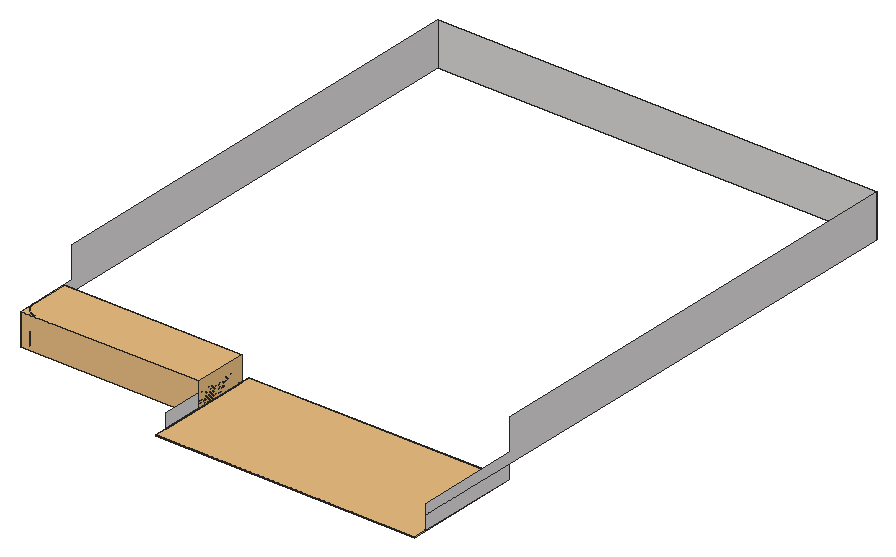
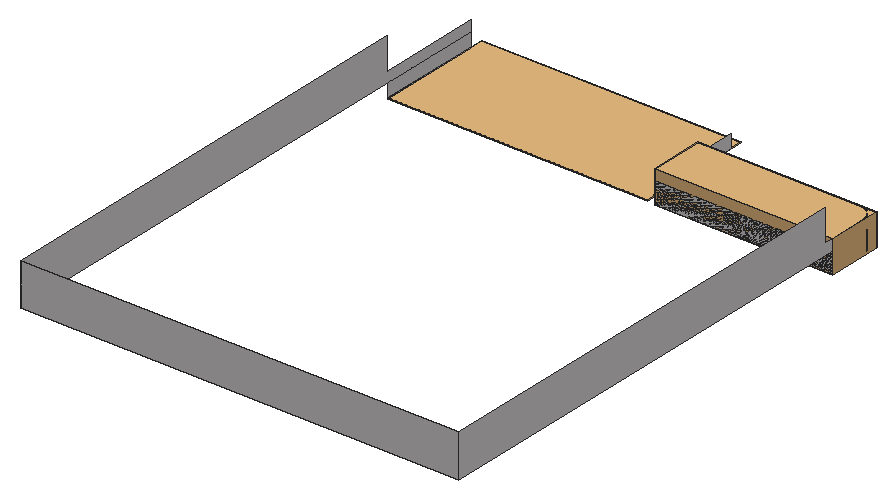
# SketchUp Ruby script. Lengths in inches.
U = 1.inch
M = Sketchup.active_model
def pt(a) = Geom::Point3d.new(a.map { |v| v * U })
def face(e, loops, mat)
  f = e.add_face(loops[0].map { |a| pt(a) })
  loops[1..].each { |l| e.add_face(l.map { |a| pt(a) }).erase! }
  f.material = f.back_material = mat if mat
  f
end
# faces: each face lists its corners as indices into pts; further lists are holes
def faces(e, pts, list, mat = nil) = list.each { |f| face(e, (f[0].is_a?(Array) ? f : [f]).map { |l| l.map { |i| pts[i] } }, mat) }
# xy, xz, yz: faces in a plane at the given z, y or x. An outline is a flat list of corners, or four numbers for a rectangle; further outlines are holes
def ring(l) = l.size == 4 ? [[l[0], l[1]], [l[2], l[1]], [l[2], l[3]], [l[0], l[3]]] : l.each_slice(2).to_a
def flat(e, list, mat, &to3) = list.each { |f| face(e, (f[0].is_a?(Array) ? f : [f]).map { |l| ring(l).map { |u, v| to3.(u, v) } }, mat) }
def xy(e, z, list, mat = nil) = flat(e, list, mat) { |x, y| [x, y, z] }
def xz(e, y, list, mat = nil) = flat(e, list, mat) { |x, z| [x, y, z] }
def yz(e, x, list, mat = nil) = flat(e, list, mat) { |y, z| [x, y, z] }
def lines(e, pts, list) = list.each { |a, b| e.add_line(pt(pts[a]), pt(pts[b])) }
# prism: a flat outline (further loops are holes) pulled along v
def prism(e, loops, v, mat = nil)
  f = face(e, loops, mat); d = Geom::Vector3d.new(v.map { |x| x * U })
  f.pushpull(f.normal.samedirection?(d) ? d.length : -d.length)
end
def box(e, o, s, mat = nil) = prism(e, [[o, [o[0] + s[0], o[1], o[2]], [o[0] + s[0], o[1] + s[1], o[2]], [o[0], o[1] + s[1], o[2]]]], [0, 0, s[2]], mat)
def at(x, y, z, deg = 0) = Geom::Transformation.translation(pt([x, y, z])) * Geom::Transformation.rotation(ORIGIN, Z_AXIS, deg.degrees)
def axes(o, x, y, z) = Geom::Transformation.new([*x, 0, *y, 0, *z, 0, *pt(o).to_a, 1])
def part(name) = M.definitions.add(name)
# library, detail: a bought-in or finely detailed component or shape, given as its bounding box
def library(name, o, s) = part(name).tap { |d| box(d.entities, o, s) }
def detail(e, o, s) = box(e.add_group.entities, o, s)
def put(e, d, t, mat = nil) = e.add_instance(d, t).tap { |i| i.material = mat if mat }
def group(e, t, mat = nil) = e.add_group.tap { |g| g.transformation = t; g.material = mat if mat }.entities
root = M.entities
M.materials.add("Outer Light - 1").color = [251, 216, 141]
M.materials.add("[Quartz Light Brown]").color = [215, 212, 212]
M.materials.add("[Wood Cherry Original]").color = [152, 86, 42]
c1 = library("Group\#15",[-0.75,-0.75,0],[293.5,131.75,1])
c2 = library("Group\#45",[-0.5,-0.5,0],[201.5,61.5,36])
xy(root,360,[[[17.76,205,17.53,205.01,17.29,205.01,17.06,205.02,16.82,205.04,16.59,205.06,16.35,205.08,16.12,205.1,15.88,205.125,15.65,205.15,15.42,205.1875,15.18,205.22,14.72,205.3,14.49,205.35,14.26,205.39,14.03,205.44,13.8,205.5,13.57,205.55,13.34,205.61,13.11,205.68,12.89,205.74,12.66,205.81,12.4375,205.88,12.21,205.96,11.99,206.03,11.77,206.11,11.55,206.2,11.33,206.28,10.89,206.46,10.68,206.56,10.46,206.65,10.25,206.75,10.04,206.86,9.83,206.96,9.41,207.18,9.2,207.3,9,207.41,8.6,207.65,8.39,207.78,8.2,207.9,8,208.03,7.8,208.17,7.61,208.3,7.42,208.4375,7.23,208.58,7.04,208.72,6.86,208.86,6.67,209.01,6.49,209.16,6.31,209.3125,6.13,209.47,5.96,209.625,5.78,209.78,5.61,209.94,5.44,210.11,5.27,210.27,5.11,210.44,4.94,210.61,4.78,210.78,4.625,210.96,4.47,211.13,4.3125,211.31,4.16,211.49,4.01,211.67,3.86,211.86,3.72,212.04,3.58,212.23,3.4375,212.42,3.3,212.61,3.17,212.8,3.03,213,2.9,213.2,2.78,213.39,2.65,213.6,2.41,214,2.3,214.2,2.18,214.41,1.96,214.83,1.86,215.04,1.75,215.25,1.65,215.46,1.56,215.68,1.46,215.89,1.28,216.33,1.2,216.55,1.11,216.77,1.03,216.99,0.96,217.21,0.88,217.4375,0.81,217.66,0.74,217.89,0.68,218.11,0.61,218.34,0.55,218.57,0.5,218.8,0.44,219.03,0.39,219.26,0.35,219.49,0.3,219.72,0.22,220.18,0.1875,220.42,0.15,220.65,0.125,220.88,0.1,221.12,0.08,221.35,0.06,221.59,0.04,221.82,0.02,222.06,0.01,222.29,0.01,222.53,0,222.76,0,266,201,266,201,205],[17.79,207,199,207,199,264,2,264,2,222.79,2.01,222.58,2.01,222.37,2.03,221.95,2.05,221.74,2.07,221.54,2.11,221.12,2.17,220.7,2.2,220.5,2.23,220.29,2.27,220.08,2.31,219.88,2.35,219.67,2.39,219.47,2.44,219.26,2.49,219.0625,2.55,218.86,2.6,218.66,2.78,218.06,2.99,217.46,3.0625,217.27,3.14,217.07,3.22,216.88,3.3,216.68,3.38,216.49,3.65,215.92,3.74,215.74,3.84,215.55,3.9375,215.37,4.04,215.18,4.14,215,4.47,214.46,4.58,214.29,4.7,214.11,4.8125,213.9375,4.93,213.77,5.06,213.6,5.18,213.43,5.31,213.26,5.43,213.09,5.57,212.93,5.83,212.61,6.11,212.29,6.39,211.99,6.54,211.84,6.6875,211.6875,6.84,211.54,6.99,211.39,7.29,211.11,7.61,210.83,7.93,210.57,8.09,210.43,8.26,210.31,8.43,210.18,8.6,210.06,8.77,209.93,8.9375,209.8125,9.11,209.7,9.29,209.58,9.46,209.47,10,209.14,10.18,209.04,10.37,208.9375,10.55,208.84,10.74,208.74,10.92,208.65,11.49,208.38,11.68,208.3,11.88,208.22,12.07,208.14,12.27,208.0625,12.46,207.99,13.06,207.78,13.66,207.6,13.86,207.55,14.0625,207.49,14.26,207.44,14.47,207.39,14.67,207.35,14.88,207.31,15.08,207.27,15.29,207.23,15.5,207.2,15.7,207.17,16.12,207.11,16.54,207.07,16.74,207.05,16.95,207.03,17.37,207.01,17.58,207.01]]],"[Quartz Light Brown]")
xy(root,366,[[17.79,207,17.58,207.01,17.37,207.01,16.95,207.03,16.74,207.05,16.54,207.07,16.12,207.11,15.7,207.17,15.5,207.2,15.29,207.23,15.08,207.27,14.88,207.31,14.67,207.35,14.47,207.39,14.26,207.44,14.0625,207.49,13.86,207.55,13.66,207.6,13.06,207.78,12.46,207.99,12.27,208.0625,12.07,208.14,11.88,208.22,11.68,208.3,11.49,208.38,10.92,208.65,10.74,208.74,10.55,208.84,10.37,208.9375,10.18,209.04,10,209.14,9.46,209.47,9.29,209.58,9.11,209.7,8.9375,209.8125,8.77,209.93,8.6,210.06,8.43,210.18,8.26,210.31,8.09,210.43,7.93,210.57,7.61,210.83,7.29,211.11,6.99,211.39,6.84,211.54,6.6875,211.6875,6.54,211.84,6.39,211.99,6.11,212.29,5.83,212.61,5.57,212.93,5.43,213.09,5.31,213.26,5.18,213.43,5.06,213.6,4.93,213.77,4.8125,213.9375,4.7,214.11,4.58,214.29,4.47,214.46,4.14,215,4.04,215.18,3.9375,215.37,3.84,215.55,3.74,215.74,3.65,215.92,3.38,216.49,3.3,216.68,3.22,216.88,3.14,217.07,3.0625,217.27,2.99,217.46,2.78,218.06,2.6,218.66,2.55,218.86,2.49,219.0625,2.44,219.26,2.39,219.47,2.35,219.67,2.31,219.88,2.27,220.08,2.23,220.29,2.2,220.5,2.17,220.7,2.11,221.12,2.07,221.54,2.05,221.74,2.03,221.95,2.01,222.37,2.01,222.58,2,222.79,2,264,199,264,199,207]],"[Quartz Light Brown]")
xz(root,207,[[17.79,360,18,366],[18,360,199,366]],"[Quartz Light Brown]")
xz(root,207.01,[[17.37,360,17.58,366]],"[Quartz Light Brown]")
xz(root,264,[[2,360,199,366]],"[Quartz Light Brown]")
xz(root,266,[[0,360,201,384]],"[Quartz Light Brown]")
xz(root,794,[[0,384,495,432]],"[Quartz Light Brown]")
yz(root,0,[[222.76,360,223,396],[223,360,266,396],[266,384,266,396,276.5,396,276.5,432,794,432,794,384]],"[Quartz Light Brown]")
yz(root,0.01,[[222.29,360,222.53,396]],"[Quartz Light Brown]")
yz(root,2,[[222.79,360,223,366],[223,360,264,366]],"[Quartz Light Brown]")
yz(root,2.01,[[222.37,360,222.58,366]],"[Quartz Light Brown]")
yz(root,199,[[207,360,264,366]],"[Quartz Light Brown]")
yz(root,201,[[205,360,266,384],[158,369,266,384]],"[Quartz Light Brown]")
yz(root,202,[[158,368,266,369]],"[Quartz Light Brown]")
yz(root,494,[[158,368,275,369]],"[Quartz Light Brown]")
yz(root,495,[[158,369,275,384],[158,384,794,384,794,432,276.5,432,276.5,396,158,396]],"[Quartz Light Brown]")
p = [[15.18,205.22,396],[14.95,205.26,396],[14.95,205.26,360],[15.18,205.22,360],[15.42,205.1875,396],[15.42,205.1875,360],
  [14.49,205.35,396],[14.26,205.39,396],[14.26,205.39,360],[14.49,205.35,360],[14.72,205.3,396],[14.72,205.3,360],
  [14.03,205.44,396],[13.8,205.5,396],[13.8,205.5,360],[14.03,205.44,360],[13.57,205.55,396],[13.57,205.55,360],
  [13.34,205.61,396],[13.11,205.68,396],[13.11,205.68,360],[13.34,205.61,360],[12.89,205.74,396],[12.66,205.81,396],
  [12.66,205.81,360],[12.89,205.74,360],[12.4375,205.88,396],[12.4375,205.88,360],[12.21,205.96,396],[12.21,205.96,360],
  [11.99,206.03,396],[11.77,206.11,396],[11.77,206.11,360],[11.99,206.03,360],[11.55,206.2,396],[11.55,206.2,360],
  [11.33,206.28,396],[11.33,206.28,360],[11.11,206.37,396],[11.11,206.37,360],[10.89,206.46,396],[10.89,206.46,360],
  [10.68,206.56,396],[10.68,206.56,360],[10.46,206.65,396],[10.46,206.65,360],[10.25,206.75,396],[10.25,206.75,360],
  [10.04,206.86,396],[10.04,206.86,360],[9.83,206.96,396],[9.83,206.96,360],[9.62,207.07,396],[9.62,207.07,360],
  [16.74,207.05,360],[16.54,207.07,360],[16.54,207.07,366],[16.74,207.05,366],[16.95,207.03,360],[16.95,207.03,366],
  [17.16,207.02,360],[17.16,207.02,366],[17.37,207.01,360],[17.37,207.01,366],[17.79,207,360],[17.58,207.01,360],
  [17.58,207.01,366],[17.79,207,366],[9.41,207.18,396],[9.41,207.18,360],[15.91,207.14,360],[15.7,207.17,360],
  [15.7,207.17,366],[15.91,207.14,366],[16.12,207.11,360],[16.12,207.11,366],[16.33,207.09,360],[16.33,207.09,366],
  [9.2,207.3,396],[9.2,207.3,360],[15.29,207.23,360],[15.08,207.27,360],[15.08,207.27,366],[15.29,207.23,366],
  [15.5,207.2,360],[15.5,207.2,366],[9,207.41,396],[9,207.41,360],[14.67,207.35,360],[14.47,207.39,360],
  [14.47,207.39,366],[14.67,207.35,366],[14.88,207.31,360],[14.88,207.31,366],[8.8,207.53,396],[8.8,207.53,360],
  [14.26,207.44,360],[14.0625,207.49,360],[14.0625,207.49,366],[14.26,207.44,366],[8.6,207.65,396],[8.6,207.65,360],
  [13.86,207.55,360],[13.66,207.6,360],[13.66,207.6,366],[13.86,207.55,366],[13.46,207.66,360],[13.46,207.66,366],
  [8.39,207.78,396],[8.39,207.78,360],[13.26,207.72,360],[13.06,207.78,360],[13.06,207.78,366],[13.26,207.72,366],
  [8.2,207.9,396],[8.2,207.9,360],[12.86,207.85,360],[12.66,207.92,360],[12.66,207.92,366],[12.86,207.85,366],
  [8,208.03,396],[8,208.03,360],[12.46,207.99,360],[12.46,207.99,366],[7.8,208.17,396],[7.8,208.17,360],
  [12.27,208.0625,360],[12.27,208.0625,366],[12.07,208.14,360],[11.88,208.22,360],[11.88,208.22,366],[12.07,208.14,366],
  [7.61,208.3,396],[7.61,208.3,360],[11.68,208.3,360],[11.68,208.3,366],[7.42,208.4375,396],[7.42,208.4375,360],
  [11.49,208.38,360],[11.49,208.38,366],[7.23,208.58,396],[7.23,208.58,360],[11.3,208.47,360],[11.3,208.47,366],
  [11.11,208.56,360],[11.11,208.56,366],[7.04,208.72,396],[7.04,208.72,360],[10.92,208.65,360],[10.92,208.65,366],
  [6.86,208.86,396],[6.86,208.86,360],[10.74,208.74,360],[10.55,208.84,360],[10.55,208.84,366],[10.74,208.74,366],
  [10.37,208.9375,360],[10.37,208.9375,366],[6.67,209.01,396],[6.67,209.01,360],[10.18,209.04,360],[10.18,209.04,366],
  [6.49,209.16,396],[6.49,209.16,360],[10,209.14,360],[10,209.14,366],[9.82,209.25,360],[9.82,209.25,366],
  [6.31,209.3125,396],[6.31,209.3125,360],[9.64,209.36,360],[9.64,209.36,366],[6.13,209.47,396],[6.13,209.47,360],
  [9.46,209.47,360],[9.46,209.47,366],[5.96,209.625,396],[5.96,209.625,360],[9.29,209.58,360],[9.29,209.58,366],
  [5.78,209.78,396],[5.78,209.78,360],[9.11,209.7,360],[9.11,209.7,366],[8.9375,209.8125,360],[8.9375,209.8125,366],
  [5.61,209.94,396],[5.61,209.94,360],[8.77,209.93,360],[8.77,209.93,366],[5.44,210.11,396],[5.44,210.11,360],
  [8.6,210.06,360],[8.6,210.06,366],[5.27,210.27,396],[5.27,210.27,360],[8.43,210.18,360],[8.43,210.18,366],
  [8.26,210.31,360],[8.26,210.31,366],[5.11,210.44,396],[5.11,210.44,360],[8.09,210.43,360],[8.09,210.43,366],
  [4.94,210.61,396],[4.94,210.61,360],[7.93,210.57,360],[7.93,210.57,366],[4.78,210.78,396],[4.78,210.78,360],
  [7.77,210.7,360],[7.77,210.7,366],[7.61,210.83,360],[7.61,210.83,366],[4.625,210.96,396],[4.625,210.96,360],
  [7.45,210.97,360],[7.45,210.97,366],[4.47,211.13,396],[4.47,211.13,360],[7.29,211.11,360],[7.29,211.11,366],
  [4.3125,211.31,396],[4.3125,211.31,360],[7.14,211.25,360],[7.14,211.25,366],[4.16,211.49,396],[4.16,211.49,360],
  [6.99,211.39,360],[6.99,211.39,366],[6.84,211.54,360],[6.84,211.54,366],[4.01,211.67,396],[4.01,211.67,360],
  [6.6875,211.6875,360],[6.6875,211.6875,366],[3.86,211.86,396],[3.86,211.86,360],[6.54,211.84,360],[6.54,211.84,366],
  [6.39,211.99,360],[6.39,211.99,366],[3.72,212.04,396],[3.72,212.04,360],[3.58,212.23,396],[3.58,212.23,360],
  [6.25,212.14,360],[6.25,212.14,366],[6.11,212.29,360],[6.11,212.29,366],[3.4375,212.42,396],[3.4375,212.42,360],
  [5.97,212.45,360],[5.97,212.45,366],[3.3,212.61,396],[3.3,212.61,360],[5.83,212.61,360],[5.83,212.61,366],
  [3.17,212.8,396],[3.17,212.8,360],[5.7,212.77,360],[5.7,212.77,366],[3.03,213,396],[3.03,213,360],
  [5.57,212.93,360],[5.57,212.93,366],[5.43,213.09,360],[5.43,213.09,366],[2.9,213.2,396],[2.9,213.2,360],
  [5.31,213.26,360],[5.31,213.26,366],[2.78,213.39,396],[2.78,213.39,360],[5.18,213.43,360],[5.18,213.43,366],
  [2.65,213.6,396],[2.65,213.6,360],[5.06,213.6,360],[5.06,213.6,366],[2.53,213.8,396],[2.53,213.8,360],
  [4.93,213.77,360],[4.93,213.77,366],[2.41,214,396],[2.41,214,360],[4.8125,213.9375,360],[4.8125,213.9375,366],
  [4.7,214.11,360],[4.7,214.11,366],[2.3,214.2,396],[2.3,214.2,360],[4.58,214.29,360],[4.58,214.29,366],
  [2.18,214.41,396],[2.18,214.41,360],[4.47,214.46,360],[4.47,214.46,366],[2.07,214.62,396],[2.07,214.62,360],
  [4.36,214.64,360],[4.36,214.64,366],[1.96,214.83,396],[1.96,214.83,360],[4.25,214.82,360],[4.25,214.82,366],
  [1.86,215.04,396],[1.86,215.04,360],[4.14,215,360],[4.14,215,366],[1.75,215.25,396],[1.75,215.25,360],
  [4.04,215.18,360],[4.04,215.18,366],[3.9375,215.37,360],[3.9375,215.37,366],[1.65,215.46,396],[1.65,215.46,360],
  [3.84,215.55,360],[3.84,215.55,366],[1.56,215.68,396],[1.56,215.68,360],[3.74,215.74,360],[3.74,215.74,366],
  [1.46,215.89,396],[1.46,215.89,360],[3.65,215.92,360],[3.65,215.92,366],[1.37,216.11,396],[1.37,216.11,360],
  [3.56,216.11,360],[3.56,216.11,366],[1.28,216.33,396],[1.28,216.33,360],[3.47,216.3,360],[3.47,216.3,366],
  [1.2,216.55,396],[1.2,216.55,360],[3.38,216.49,360],[3.38,216.49,366],[1.11,216.77,396],[1.11,216.77,360],
  [3.3,216.68,360],[3.3,216.68,366],[3.22,216.88,360],[3.22,216.88,366],[1.03,216.99,396],[1.03,216.99,360],
  [3.14,217.07,360],[3.14,217.07,366],[0.96,217.21,396],[0.96,217.21,360],[3.0625,217.27,360],[3.0625,217.27,366],
  [0.88,217.4375,396],[0.88,217.4375,360],[2.99,217.46,360],[2.99,217.46,366],[0.81,217.66,396],[0.81,217.66,360],
  [2.92,217.66,360],[2.92,217.66,366],[0.74,217.89,396],[0.74,217.89,360],[2.85,217.86,360],[2.85,217.86,366],
  [0.68,218.11,396],[0.68,218.11,360],[2.78,218.06,360],[2.78,218.06,366],[0.61,218.34,396],[0.61,218.34,360],
  [2.72,218.26,360],[2.72,218.26,366],[0.55,218.57,396],[0.55,218.57,360],[2.66,218.46,360],[2.66,218.46,366],
  [2.6,218.66,360],[2.6,218.66,366],[0.5,218.8,396],[0.5,218.8,360],[2.55,218.86,360],[2.55,218.86,366],
  [0.44,219.03,396],[0.44,219.03,360],[2.49,219.0625,360],[2.49,219.0625,366],[0.39,219.26,396],[0.39,219.26,360],
  [2.44,219.26,360],[2.44,219.26,366],[0.35,219.49,396],[0.35,219.49,360],[2.39,219.47,360],[2.39,219.47,366],
  [0.3,219.72,396],[0.3,219.72,360],[2.35,219.67,360],[2.35,219.67,366],[0.26,219.95,396],[0.26,219.95,360],
  [2.31,219.88,360],[2.31,219.88,366],[2.27,220.08,360],[2.27,220.08,366],[0.22,220.18,396],[0.22,220.18,360],
  [2.23,220.29,360],[2.23,220.29,366],[0.1875,220.42,396],[0.1875,220.42,360],[2.2,220.5,360],[2.2,220.5,366],
  [0.15,220.65,396],[0.15,220.65,360],[2.17,220.7,360],[2.17,220.7,366],[0.125,220.88,396],[0.125,220.88,360],
  [2.14,220.91,360],[2.14,220.91,366],[0.1,221.12,396],[0.1,221.12,360],[2.11,221.12,360],[2.11,221.12,366],
  [0.08,221.35,396],[0.08,221.35,360],[2.09,221.33,360],[2.09,221.33,366],[2.07,221.54,360],[2.07,221.54,366],
  [0.06,221.59,396],[0.06,221.59,360],[2.05,221.74,360],[2.05,221.74,366],[0.04,221.82,396],[0.04,221.82,360],
  [2.03,221.95,360],[2.03,221.95,366],[0.02,222.06,396],[0.02,222.06,360],[2.02,222.16,360],[2.02,222.16,366],
  [0.01,222.29,396],[0.01,222.29,360],[2.01,222.37,360],[2.01,222.37,366],[0.01,222.53,396],[0,222.76,396],
  [0,222.76,360],[0.01,222.53,360],[2.01,222.58,360],[2,222.79,360],[2,222.79,366],[2.01,222.58,366]]
faces(root,p,[[0,1,2,3],[4,0,3,5],[6,7,8,9],[10,6,9,11],[1,10,11,2],[12,13,14,15],[7,12,15,8],[13,16,17,14],
  [18,19,20,21],[16,18,21,17],[22,23,24,25],[19,22,25,20],[23,26,27,24],[26,28,29,27],[30,31,32,33],[28,30,33,29],
  [31,34,35,32],[34,36,37,35],[36,38,39,37],[38,40,41,39],[40,42,43,41],[42,44,45,43],[44,46,47,45],[46,48,49,47],
  [48,50,51,49],[50,52,53,51],[54,55,56,57],[58,54,57,59],[60,58,59,61],[62,60,61,63],[64,65,66,67],[52,68,69,53],
  [70,71,72,73],[74,70,73,75],[76,74,75,77],[55,76,77,56],[68,78,79,69],[80,81,82,83],[84,80,83,85],[71,84,85,72],
  [78,86,87,79],[88,89,90,91],[92,88,91,93],[81,92,93,82],[86,94,95,87],[96,97,98,99],[89,96,99,90],[94,100,101,95],
  [102,103,104,105],[97,102,105,98],[103,106,107,104],[100,108,109,101],[110,111,112,113],[106,110,113,107],[108,114,115,109],[116,117,118,119],
  [111,116,119,112],[114,120,121,115],[117,122,123,118],[120,124,125,121],[122,126,127,123],[128,129,130,131],[126,128,131,127],[124,132,133,125],
  [129,134,135,130],[132,136,137,133],[134,138,139,135],[136,140,141,137],[138,142,143,139],[142,144,145,143],[140,146,147,141],[144,148,149,145],
  [146,150,151,147],[152,153,154,155],[148,152,155,149],[153,156,157,154],[150,158,159,151],[156,160,161,157],[158,162,163,159],[160,164,165,161],
  [164,166,167,165],[162,168,169,163],[166,170,171,167],[168,172,173,169],[170,174,175,171],[172,176,177,173],[174,178,179,175],[176,180,181,177],
  [178,182,183,179],[182,184,185,183],[180,186,187,181],[184,188,189,185],[186,190,191,187],[188,192,193,189],[190,194,195,191],[192,196,197,193],
  [196,198,199,197],[194,200,201,195],[198,202,203,199],[200,204,205,201],[202,206,207,203],[204,208,209,205],[206,210,211,207],[210,212,213,211],
  [208,214,215,209],[212,216,217,213],[214,218,219,215],[216,220,221,217],[218,222,223,219],[220,224,225,221],[222,226,227,223],[224,228,229,225],
  [228,230,231,229],[226,232,233,227],[230,234,235,231],[232,236,237,233],[234,238,239,235],[238,240,241,239],[236,242,243,237],[242,244,245,243],
  [240,246,247,241],[246,248,249,247],[244,250,251,245],[248,252,253,249],[250,254,255,251],[252,256,257,253],[254,258,259,255],[256,260,261,257],
  [258,262,263,259],[260,264,265,261],[264,266,267,265],[262,268,269,263],[266,270,271,267],[268,272,273,269],[270,274,275,271],[272,276,277,273],
  [274,278,279,275],[276,280,281,277],[278,282,283,279],[280,284,285,281],[282,286,287,283],[286,288,289,287],[284,290,291,285],[288,292,293,289],
  [290,294,295,291],[292,296,297,293],[294,298,299,295],[296,300,301,297],[298,302,303,299],[300,304,305,301],[302,306,307,303],[304,308,309,305],
  [306,310,311,307],[308,312,313,309],[312,314,315,313],[310,316,317,311],[314,318,319,315],[316,320,321,317],[318,322,323,319],[320,324,325,321],
  [322,326,327,323],[324,328,329,325],[326,330,331,327],[328,332,333,329],[330,334,335,331],[332,336,337,333],[334,338,339,335],[336,340,341,337],
  [338,342,343,339],[342,344,345,343],[340,346,347,341],[344,348,349,345],[346,350,351,347],[348,352,353,349],[350,354,355,351],[352,356,357,353],
  [354,358,359,355],[356,360,361,357],[358,362,363,359],[360,364,365,361],[362,366,367,363],[364,368,369,365],[366,370,371,367],[368,372,373,369],
  [370,374,375,371],[372,376,377,373],[376,378,379,377],[374,380,381,375],[378,382,383,379],[380,384,385,381],[382,386,387,383],[384,388,389,385],
  [386,390,391,387],[388,392,393,389],[390,394,395,391],[392,396,397,393],[394,398,399,395],[396,400,401,397],[398,402,403,399],[402,404,405,403],
  [400,406,407,401],[404,408,409,405],[406,410,411,407],[408,412,413,409],[410,414,415,411],[412,416,417,413],[414,418,419,415],[416,420,421,417],
  [418,422,423,419],[420,424,425,421],[422,426,427,423],[424,428,429,425],[428,430,431,429],[426,432,433,427],[430,434,435,431],[432,436,437,433],
  [434,438,439,435],[436,440,441,437],[438,442,443,439],[440,444,445,441],[442,446,447,443],[448,449,450,451],[452,453,454,455]],"[Quartz Light Brown]")
put(root,c1,at(202,144,368),"Outer Light - 1")
put(root,c2,at(0,205,360),"[Wood Cherry Original]")
